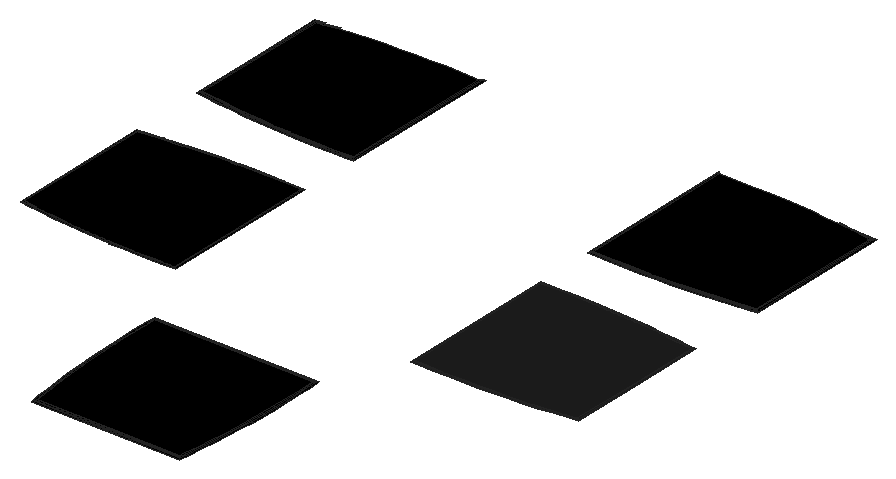
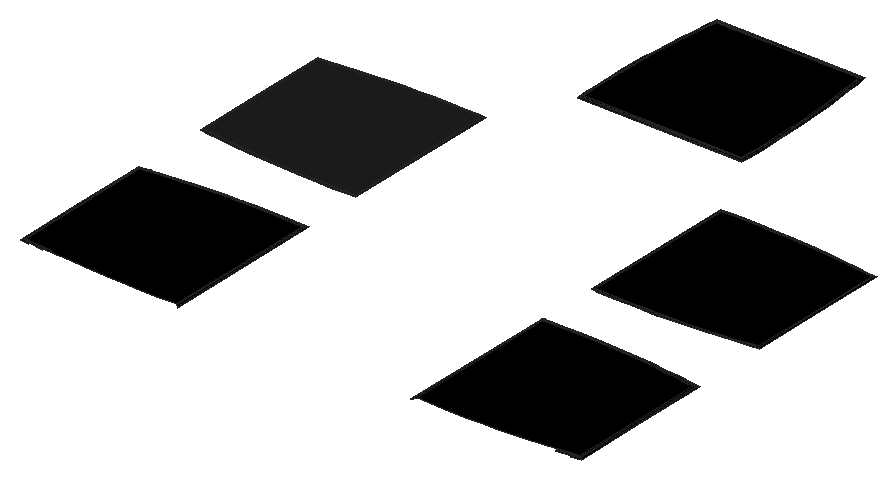
# SketchUp Ruby script. Lengths in inches.
U = 1.inch
M = Sketchup.active_model
def pt(a) = Geom::Point3d.new(a.map { |v| v * U })
def face(e, loops, mat)
  f = e.add_face(loops[0].map { |a| pt(a) })
  loops[1..].each { |l| e.add_face(l.map { |a| pt(a) }).erase! }
  f.material = f.back_material = mat if mat
  f
end
# faces: each face lists its corners as indices into pts; further lists are holes
def faces(e, pts, list, mat = nil) = list.each { |f| face(e, (f[0].is_a?(Array) ? f : [f]).map { |l| l.map { |i| pts[i] } }, mat) }
# xy, xz, yz: faces in a plane at the given z, y or x. An outline is a flat list of corners, or four numbers for a rectangle; further outlines are holes
def ring(l) = l.size == 4 ? [[l[0], l[1]], [l[2], l[1]], [l[2], l[3]], [l[0], l[3]]] : l.each_slice(2).to_a
def flat(e, list, mat, &to3) = list.each { |f| face(e, (f[0].is_a?(Array) ? f : [f]).map { |l| ring(l).map { |u, v| to3.(u, v) } }, mat) }
def xy(e, z, list, mat = nil) = flat(e, list, mat) { |x, y| [x, y, z] }
def xz(e, y, list, mat = nil) = flat(e, list, mat) { |x, z| [x, y, z] }
def yz(e, x, list, mat = nil) = flat(e, list, mat) { |y, z| [x, y, z] }
def lines(e, pts, list) = list.each { |a, b| e.add_line(pt(pts[a]), pt(pts[b])) }
# prism: a flat outline (further loops are holes) pulled along v
def prism(e, loops, v, mat = nil)
  f = face(e, loops, mat); d = Geom::Vector3d.new(v.map { |x| x * U })
  f.pushpull(f.normal.samedirection?(d) ? d.length : -d.length)
end
def box(e, o, s, mat = nil) = prism(e, [[o, [o[0] + s[0], o[1], o[2]], [o[0] + s[0], o[1] + s[1], o[2]], [o[0], o[1] + s[1], o[2]]]], [0, 0, s[2]], mat)
def at(x, y, z, deg = 0) = Geom::Transformation.translation(pt([x, y, z])) * Geom::Transformation.rotation(ORIGIN, Z_AXIS, deg.degrees)
def axes(o, x, y, z) = Geom::Transformation.new([*x, 0, *y, 0, *z, 0, *pt(o).to_a, 1])
def part(name) = M.definitions.add(name)
# library, detail: a bought-in or finely detailed component or shape, given as its bounding box
def library(name, o, s) = part(name).tap { |d| box(d.entities, o, s) }
def detail(e, o, s) = box(e.add_group.entities, o, s)
def put(e, d, t, mat = nil) = e.add_instance(d, t).tap { |i| i.material = mat if mat }
def group(e, t, mat = nil) = e.add_group.tap { |g| g.transformation = t; g.material = mat if mat }.entities
root = M.entities
M.materials.add("[Color M08]").color = [30, 30, 30]
M.materials.add("[Color M09]").color = [0, 0, 0]
xy(root,29.97,[[132.31,88.17,134,88.18,135.68,88.23,135.7,88.23,137.375,88.3,139.0625,88.39,140.75,88.52,142.43,88.68,144.1,88.86,145.78,89.07,146.49,89.17,146.49,105.6,145.78,105.7,144.1,105.91,142.43,106.09,140.75,106.24,139.0625,106.37,137.375,106.47,135.7,106.54,135.68,106.54,134,106.58,132.31,106.59,130.625,106.58,128.9375,106.54,128.32,106.51,128.32,88.25,128.9375,88.23,130.625,88.18]],"[Color M08]")
xy(root,29.97,[[106.15,61.21,122.58,61.21,122.68,61.92,122.89,63.6,123.07,65.28,123.22,66.96,123.35,68.64,123.45,70.33,123.52,72,123.52,72.02,123.56,73.7,123.57,75.39,123.56,77.08,123.52,78.76,123.49,79.38,105.23,79.38,105.21,78.76,105.16,77.08,105.15,75.39,105.16,73.7,105.21,72.02,105.21,72,105.28,70.33,105.375,68.64,105.5,66.96,105.65,65.28,105.84,63.6,106.05,61.92],[96.41,88.17,98.1,88.18,99.78,88.23,100.4,88.25,100.4,106.51,99.78,106.54,98.1,106.58,96.41,106.59,94.72,106.58,93.04,106.54,93.02,106.54,91.35,106.47,89.66,106.37,87.98,106.24,86.3,106.09,84.62,105.91,82.94,105.7,82.23,105.6,82.23,89.17,82.94,89.07,84.62,88.86,86.3,88.68,87.98,88.52,89.66,88.39,91.35,88.3,93.02,88.23,93.04,88.23,94.72,88.18],[96.41,114.08,98.1,114.09,99.78,114.13,100.4,114.16,100.4,132.42,99.78,132.44,98.1,132.49,96.41,132.5,94.72,132.49,93.04,132.44,93.02,132.44,91.35,132.375,89.66,132.28,87.98,132.15,86.3,132,84.62,131.8125,82.94,131.6,82.23,131.5,82.23,115.07,82.94,114.97,84.62,114.76,86.3,114.58,87.98,114.43,89.66,114.3,91.35,114.2,93.02,114.13,93.04,114.13,94.72,114.09],[132.31,114.08,134,114.09,135.68,114.13,135.7,114.13,137.375,114.2,139.0625,114.3,140.75,114.43,142.43,114.58,144.1,114.76,145.78,114.97,146.49,115.07,146.49,131.5,145.78,131.6,144.1,131.8125,142.43,132,140.75,132.15,139.0625,132.28,137.375,132.375,135.7,132.44,135.68,132.44,134,132.49,132.31,132.5,130.625,132.49,128.9375,132.44,128.32,132.42,128.32,114.16,128.9375,114.13,130.625,114.09]],"[Color M09]")
p = [[105.76,61.89,29.93],[105.62,61.87,29.89],[105.77,60.78,29.89],[105.9,60.92,29.93],[114.36,60.78,29.89],[114.36,60.92,29.93],
  [122.95,60.78,29.89],[122.83,60.92,29.93],[123.1,61.87,29.89],[122.97,61.89,29.93],[105.9,61.9,29.96],[106.02,61.0625,29.96],
  [114.36,61.0625,29.96],[122.7,61.0625,29.96],[122.82,61.9,29.96],[105.55,63.57,29.93],[105.41,63.55,29.89],[105.69,63.58,29.96],
  [123.18,63.57,29.93],[123.03,63.58,29.96],[123.3125,63.55,29.89],[105.37,65.25,29.93],[105.23,65.23,29.89],[123.5,65.23,29.89],
  [123.36,65.25,29.93],[105.51,65.26,29.96],[123.21,65.26,29.96],[105.21,66.93,29.93],[105.07,66.92,29.89],[105.35,66.95,29.96],
  [123.51,66.93,29.93],[123.37,66.95,29.96],[123.65,66.92,29.89],[105.08,68.62,29.93],[104.94,68.61,29.89],[105.23,68.63,29.96],
  [123.64,68.62,29.93],[123.5,68.63,29.96],[123.78,68.61,29.89],[104.99,70.3125,29.93],[104.85,70.31,29.89],[105.13,70.32,29.96],
  [123.74,70.3125,29.93],[123.59,70.32,29.96],[123.88,70.31,29.89],[104.78,71.99,29.89],[104.91,72,29.93],[105.06,72,29.96],
  [123.81,72,29.93],[123.66,72,29.96],[123.95,71.99,29.89],[104.78,72.01,29.89],[104.73,73.69,29.89],[104.87,73.7,29.93],
  [104.91,72.01,29.93],[105.06,72.02,29.96],[105.02,73.7,29.96],[123.67,72.02,29.96],[123.81,72.01,29.93],[123.85,73.7,29.93],
  [123.71,73.7,29.96],[123.95,72.01,29.89],[123.99,73.69,29.89],[104.72,75.39,29.89],[104.86,75.39,29.93],[105,75.39,29.96],
  [123.72,75.39,29.96],[123.87,75.39,29.93],[124,75.39,29.89],[104.73,77.08,29.89],[104.87,77.08,29.93],[105.02,77.08,29.96],
  [123.71,77.08,29.96],[123.85,77.08,29.93],[123.99,77.08,29.89],[104.77,78.78,29.89],[104.91,78.77,29.93],[105.06,78.77,29.96],
  [123.67,78.77,29.96],[123.81,78.77,29.93],[123.95,78.78,29.89],[104.82,79.8125,29.89],[104.95,79.67,29.93],[105.09,79.53,29.96],
  [123.63,79.53,29.96],[123.77,79.67,29.93],[123.91,79.8125,29.89],[91.33,88.01,29.93],[93.02,87.94,29.93],[93.02,88.08,29.96],
  [91.34,88.15,29.96],[94.72,87.89,29.93],[93.03,87.93,29.93],[93.04,88.08,29.96],[94.72,88.04,29.96],[96.41,88.02,29.96],
  [96.41,87.88,29.93],[98.1,88.04,29.96],[98.1,87.89,29.93],[99.79,88.08,29.96],[99.79,87.93,29.93],[100.55,88.11,29.96],
  [100.69,87.97,29.93],[128.93,88.08,29.96],[128.93,87.93,29.93],[128.03,87.97,29.93],[128.18,88.11,29.96],[130.625,88.04,29.96],
  [130.62,87.89,29.93],[132.31,88.02,29.96],[132.31,87.88,29.93],[134.01,88.04,29.96],[134.01,87.89,29.93],[135.69,87.93,29.93],
  [135.6875,88.08,29.96],[135.7,88.08,29.96],[135.71,87.94,29.93],[137.39,88.01,29.93],[137.38,88.15,29.96],[89.65,88.25,29.96],
  [89.64,88.1,29.93],[100.55,106.65,29.96],[100.69,106.79,29.93],[128.03,106.79,29.93],[128.18,106.65,29.96],[139.08,88.1,29.93],
  [139.07,88.25,29.96],[87.97,88.375,29.96],[87.95,88.23,29.93],[140.77,88.23,29.93],[140.76,88.375,29.96],[86.28,88.53,29.96],
  [86.27,88.39,29.93],[142.46,88.39,29.93],[142.44,88.53,29.96],[84.6,88.71,29.96],[84.59,88.57,29.93],[144.14,88.57,29.93],
  [144.12,88.71,29.96],[82.92,88.92,29.96],[82.91,88.78,29.93],[145.82,88.78,29.93],[145.8,88.92,29.96],[82.08,89.04,29.96],
  [81.9375,88.92,29.93],[146.78,88.92,29.93],[146.64,89.04,29.96],[82.08,97.38,29.96],[81.9375,97.38,29.93],[146.78,97.38,29.93],
  [146.64,97.38,29.96],[82.08,105.72,29.96],[81.9375,105.85,29.93],[146.78,105.85,29.93],[146.64,105.72,29.96],[82.92,105.84,29.96],
  [82.91,105.99,29.93],[145.82,105.99,29.93],[145.8,105.84,29.96],[84.6,106.05,29.96],[84.59,106.2,29.93],[144.14,106.2,29.93],
  [144.12,106.05,29.96],[86.28,106.24,29.96],[86.27,106.38,29.93],[142.46,106.38,29.93],[142.44,106.24,29.96],[87.97,106.39,29.96],
  [87.95,106.53,29.93],[140.77,106.53,29.93],[140.76,106.39,29.96],[89.65,106.52,29.96],[89.64,106.66,29.93],[139.08,106.66,29.93],
  [139.07,106.52,29.96],[91.34,106.61,29.96],[91.33,106.76,29.93],[137.39,106.76,29.93],[137.38,106.61,29.96],[93.02,106.83,29.93],
  [93.02,106.68,29.96],[135.71,106.83,29.93],[135.7,106.68,29.96],[93.04,106.6875,29.96],[93.03,106.83,29.93],[94.72,106.87,29.93],
  [94.72,106.73,29.96],[96.41,106.89,29.93],[96.41,106.74,29.96],[98.1,106.87,29.93],[98.1,106.73,29.96],[99.79,106.83,29.93],
  [99.79,106.6875,29.96],[128.93,106.83,29.93],[128.93,106.6875,29.96],[130.62,106.87,29.93],[130.625,106.73,29.96],[132.31,106.89,29.93],
  [132.31,106.74,29.96],[134.01,106.87,29.93],[134.01,106.73,29.96],[135.69,106.83,29.93],[135.6875,106.6875,29.96],[94.71,113.66,29.89],
  [94.72,113.8,29.93],[96.41,113.78,29.93],[96.41,113.65,29.89],[98.1,113.8,29.93],[98.1,113.66,29.89],[132.31,113.78,29.93],
  [132.31,113.65,29.89],[130.62,113.66,29.89],[130.62,113.8,29.93],[134.01,113.8,29.93],[134.01,113.66,29.89],[91.33,113.77,29.89],
  [93.01,113.7,29.89],[93.02,113.84,29.93],[91.33,113.91,29.93],[93.02,113.7,29.89],[93.03,113.84,29.93],[99.79,113.84,29.93],
  [99.8,113.7,29.89],[100.69,113.88,29.93],[100.83,113.74,29.89],[100.69,132.7,29.93],[100.83,132.83,29.89],[128.93,113.84,29.93],
  [128.92,113.7,29.89],[127.89,113.74,29.89],[128.03,113.88,29.93],[127.89,132.83,29.89],[128.03,132.7,29.93],[135.7,113.7,29.89],
  [135.69,113.84,29.93],[135.71,113.84,29.93],[135.71,113.7,29.89],[137.4,113.77,29.89],[137.39,113.91,29.93],[89.64,114.01,29.93],
  [89.63,113.87,29.89],[93.02,113.99,29.96],[91.34,114.06,29.96],[93.04,113.98,29.96],[94.72,113.94,29.96],[96.41,113.93,29.96],
  [98.1,113.94,29.96],[99.79,113.98,29.96],[100.55,114.02,29.96],[128.93,113.98,29.96],[128.18,114.02,29.96],[130.625,113.94,29.96],
  [132.31,113.93,29.96],[134.01,113.94,29.96],[135.6875,113.98,29.96],[135.7,113.99,29.96],[137.38,114.06,29.96],[139.09,113.87,29.89],
  [139.08,114.01,29.93],[87.95,114.14,29.93],[87.94,114,29.89],[89.65,114.15,29.96],[100.55,132.56,29.96],[128.18,132.56,29.96],
  [139.07,114.15,29.96],[140.78,114,29.89],[140.77,114.14,29.93],[86.27,114.29,29.93],[86.25,114.15,29.89],[87.97,114.28,29.96],
  [140.76,114.28,29.96],[142.47,114.15,29.89],[142.46,114.29,29.93],[86.28,114.44,29.96],[142.44,114.44,29.96],[84.59,114.47,29.93],
  [84.57,114.34,29.89],[144.15,114.34,29.89],[144.14,114.47,29.93],[82.91,114.68,29.93],[82.89,114.55,29.89],[84.6,114.62,29.96],
  [144.12,114.62,29.96],[145.84,114.55,29.89],[145.82,114.68,29.93],[81.9375,114.82,29.93],[81.8,114.7,29.89],[82.92,114.83,29.96],
  [145.8,114.83,29.96],[146.92,114.7,29.89],[146.78,114.82,29.93],[81.9375,123.29,29.93],[81.8,123.29,29.89],[82.08,114.95,29.96],
  [146.64,114.95,29.96],[146.92,123.29,29.89],[146.78,123.29,29.93],[82.08,123.29,29.96],[146.64,123.29,29.96],[81.9375,131.75,29.93],
  [81.8,131.875,29.89],[82.08,131.63,29.96],[146.78,131.75,29.93],[146.64,131.63,29.96],[146.92,131.875,29.89],[82.92,131.75,29.96],
  [82.91,131.89,29.93],[145.82,131.89,29.93],[145.8,131.75,29.96],[84.6,131.96,29.96],[84.59,132.1,29.93],[144.14,132.1,29.93],
  [144.12,131.96,29.96],[82.89,132.03,29.89],[145.84,132.03,29.89],[106.05,61.92,29.97],[106.15,61.21,29.97],[114.36,61.21,29.97],
  [122.58,61.21,29.97],[122.68,61.92,29.97],[105.84,63.6,29.97],[122.89,63.6,29.97],[105.65,65.28,29.97],[123.07,65.28,29.97],
  [105.5,66.96,29.97],[123.22,66.96,29.97],[105.375,68.64,29.97],[123.35,68.64,29.97],[105.28,70.33,29.97],[123.45,70.33,29.97],
  [105.21,72,29.97],[123.52,72,29.97],[105.16,73.7,29.97],[105.21,72.02,29.97],[123.52,72.02,29.97],[123.56,73.7,29.97],
  [105.15,75.39,29.97],[123.57,75.39,29.97],[105.16,77.08,29.97],[123.56,77.08,29.97],[105.21,78.76,29.97],[123.52,78.76,29.97],
  [105.23,79.38,29.97],[123.49,79.38,29.97],[93.04,88.23,29.97],[94.72,88.18,29.97],[96.41,88.17,29.97],[98.1,88.18,29.97],
  [99.78,88.23,29.97],[130.625,88.18,29.97],[128.9375,88.23,29.97],[132.31,88.17,29.97],[134,88.18,29.97],[135.68,88.23,29.97],
  [91.35,88.3,29.97],[89.66,88.39,29.97],[93.02,88.23,29.97],[100.4,88.25,29.97],[100.4,106.51,29.97],[128.32,88.25,29.97],
  [128.32,106.51,29.97],[135.7,88.23,29.97],[137.375,88.3,29.97],[139.0625,88.39,29.97],[87.98,88.52,29.97],[140.75,88.52,29.97],
  [86.3,88.68,29.97],[142.43,88.68,29.97],[84.62,88.86,29.97],[144.1,88.86,29.97],[82.94,89.07,29.97],[145.78,89.07,29.97],
  [82.23,89.17,29.97],[146.49,89.17,29.97],[82.23,97.38,29.97],[146.49,97.38,29.97],[82.23,105.6,29.97],[146.49,105.6,29.97],
  [82.94,105.7,29.97],[145.78,105.7,29.97],[84.62,105.91,29.97],[144.1,105.91,29.97],[86.3,106.09,29.97],[142.43,106.09,29.97],
  [87.98,106.24,29.97],[140.75,106.24,29.97],[89.66,106.37,29.97],[139.0625,106.37,29.97],[91.35,106.47,29.97],[137.375,106.47,29.97],
  [93.02,106.54,29.97],[93.04,106.54,29.97],[94.72,106.58,29.97],[98.1,106.58,29.97],[99.78,106.54,29.97],[128.9375,106.54,29.97],
  [130.625,106.58,29.97],[135.68,106.54,29.97],[134,106.58,29.97],[135.7,106.54,29.97],[96.41,106.59,29.97],[132.31,106.59,29.97],
  [93.04,114.13,29.97],[94.72,114.09,29.97],[96.41,114.08,29.97],[98.1,114.09,29.97],[99.78,114.13,29.97],[130.625,114.09,29.97],
  [128.9375,114.13,29.97],[132.31,114.08,29.97],[134,114.09,29.97],[135.68,114.13,29.97],[93.02,114.13,29.97],[91.35,114.2,29.97],
  [100.4,114.16,29.97],[100.4,132.42,29.97],[128.32,114.16,29.97],[128.32,132.42,29.97],[135.7,114.13,29.97],[137.375,114.2,29.97],
  [89.66,114.3,29.97],[139.0625,114.3,29.97],[87.98,114.43,29.97],[140.75,114.43,29.97],[86.3,114.58,29.97],[142.43,114.58,29.97],
  [84.62,114.76,29.97],[144.1,114.76,29.97],[82.94,114.97,29.97],[145.78,114.97,29.97],[82.23,115.07,29.97],[146.49,115.07,29.97],
  [82.23,123.29,29.97],[146.49,123.29,29.97],[82.23,131.5,29.97],[146.49,131.5,29.97],[82.94,131.6,29.97],[145.78,131.6,29.97],
  [84.62,131.8125,29.97],[144.1,131.8125,29.97],[142.44,132.14,29.96],[142.43,132,29.97]]
faces(root,p,[[0,1,2,3],[3,2,4,5],[6,7,5,4],[8,9,7,6],[10,0,3,11],[11,3,5,12],[7,13,12,5],[9,14,13,7],
  [15,16,1,0],[17,15,0,10],[18,19,14,9],[20,18,9,8],[21,22,16,15],[23,24,18,20],[25,21,15,17],[24,26,19,18],
  [27,28,22,21],[29,27,21,25],[30,31,26,24],[32,30,24,23],[33,34,28,27],[35,33,27,29],[36,37,31,30],[38,36,30,32],
  [39,40,34,33],[41,39,33,35],[42,43,37,36],[44,42,36,38],[45,40,39,46],[46,39,41,47],[42,48,49,43],[44,50,48,42],
  [51,52,53,54],[54,46,45,51],[55,47,46,54],[54,53,56,55],[57,49,48,58],[59,58,57,60],[58,48,50,61],[62,61,58,59],
  [53,52,63,64],[56,53,64,65],[59,60,66,67],[62,59,67,68],[64,63,69,70],[65,64,70,71],[67,66,72,73],[68,67,73,74],
  [70,69,75,76],[71,70,76,77],[73,72,78,79],[74,73,79,80],[76,75,81,82],[77,76,82,83],[79,78,84,85],[80,79,85,86],
  [83,82,85,84],[82,81,86,85],[87,88,89,90],[91,92,93,94],[93,89,88,92],[91,94,95,96],[96,95,97,98],[98,97,99,100],
  [100,99,101,102],[87,90,119,120],[121,122,102,101],[120,119,127,128],[128,127,131,132],[132,131,135,136],[136,135,139,140],[140,139,143,144],
  [144,143,147,148],[151,152,148,147],[155,156,152,151],[159,160,156,155],[163,164,160,159],[167,168,164,163],[171,172,168,167],[175,176,172,171],
  [179,176,175,180],[183,180,179,184],[184,185,186,183],[186,185,187,188],[188,187,189,190],[190,189,191,192],[192,191,122,121],[203,204,205,206],
  [206,205,207,208],[209,210,211,212],[213,214,210,209],[215,216,217,218],[203,219,220,204],[220,217,216,219],[208,207,221,222],[222,221,223,224],
  [225,226,224,223],[227,228,229,230],[230,229,231,232],[212,211,228,227],[233,214,213,234],[234,235,236,233],[236,237,238,235],[215,218,239,240],
  [218,217,241,242],[204,220,243,244],[243,241,217,220],[204,244,245,205],[205,245,246,207],[207,246,247,221],[221,247,248,223],[249,227,230,250],
  [251,212,227,249],[252,209,212,251],[253,213,209,252],[234,213,253,254],[254,255,235,234],[235,238,256,255],[238,237,257,258],[240,239,259,260],
  [218,242,261,239],[262,225,223,248],[250,230,232,263],[256,238,258,264],[258,257,265,266],[260,259,267,268],[239,261,269,259],[264,258,266,270],
  [266,265,271,272],[259,269,273,267],[270,266,272,274],[268,267,275,276],[272,271,277,278],[276,275,279,280],[267,273,281,275],[274,272,278,282],
  [278,277,283,284],[280,279,285,286],[275,281,287,279],[282,278,284,288],[284,283,289,290],[286,285,291,292],[279,287,293,285],[288,284,290,294],
  [290,289,295,296],[285,293,297,291],[294,290,296,298],[299,300,292,291],[301,299,291,297],[302,303,298,296],[304,302,296,295],[305,306,299,301],
  [307,308,303,302],[309,310,306,305],[311,312,308,307],[306,313,300,299],[314,307,302,304],[315,10,11,316],[316,11,12,317],[13,318,317,12],
  [14,319,318,13],[320,17,10,315],[19,321,319,14],[322,25,17,320],[26,323,321,19],[324,29,25,322],[31,325,323,26],[326,35,29,324],
  [37,327,325,31],[328,41,35,326],[43,329,327,37],[47,41,328,330],[43,49,331,329],[55,56,332,333],[333,330,47,55],[334,331,49,57],
  [60,57,334,335],[332,56,65,336],[60,335,337,66],[336,65,71,338],[66,337,339,72],[338,71,77,340],[72,339,341,78],[340,77,83,342],
  [78,341,343,84],[342,83,84,343],[94,93,344,345],[94,345,346,95],[95,346,347,97],[97,347,348,99],[90,354,355,119],[90,89,356,354],
  [344,356,89,93],[99,348,357,101],[358,121,101,357],[119,355,364,127],[127,364,366,131],[131,366,368,135],[135,368,370,139],[139,370,372,143],
  [143,372,374,147],[376,151,147,374],[378,155,151,376],[380,159,155,378],[382,163,159,380],[384,167,163,382],[386,171,167,384],[388,175,171,386],
  [180,175,388,390],[391,390,180,183],[183,186,392,391],[393,190,192,394],[394,192,121,358],[392,186,188,400],[400,188,190,393],[244,243,402,403],
  [244,403,404,245],[245,404,405,246],[246,405,406,247],[407,251,249,408],[409,252,251,407],[410,253,252,409],[254,253,410,411],[242,241,412,413],
  [402,412,241,243],[247,406,414,248],[415,262,248,414],[408,249,250,416],[416,250,263,417],[411,418,255,254],[255,256,419,418],[242,413,420,261],
  [419,256,264,421],[261,420,422,269],[421,264,270,423],[269,422,424,273],[423,270,274,425],[273,424,426,281],[425,274,282,427],[281,426,428,287],
  [427,282,288,429],[287,428,430,293],[429,288,294,431],[293,430,432,297],[431,294,298,433],[434,301,297,432],[303,435,433,298],[436,305,301,434],
  [308,437,435,303],[438,309,305,436],[312,439,437,308],[440,441,439,312]],"[Color M09]")
faces(root,p,[[103,104,105,106],[107,108,104,103],[109,110,108,107],[111,112,110,109],[113,112,111,114],[114,115,116,113],[116,117,118,115],[106,105,123,124],
  [118,117,125,126],[126,125,129,130],[130,129,133,134],[134,133,137,138],[138,137,141,142],[142,141,145,146],[146,145,149,150],[153,154,150,149],
  [157,158,154,153],[161,162,158,157],[165,166,162,161],[169,170,166,165],[173,174,170,169],[177,178,174,173],[177,181,182,178],[193,194,124,123],
  [195,196,194,193],[197,198,196,195],[199,200,198,197],[199,201,202,200],[202,182,181,201],[349,107,103,350],[351,109,107,349],[352,111,109,351],
  [114,111,352,353],[350,103,106,359],[359,106,124,360],[353,361,115,114],[115,118,362,361],[362,118,126,363],[363,126,130,365],[365,130,134,367],
  [367,134,138,369],[369,138,142,371],[371,142,146,373],[373,146,150,375],[154,377,375,150],[158,379,377,154],[162,381,379,158],[166,383,381,162],
  [170,385,383,166],[174,387,385,170],[178,389,387,174],[194,395,360,124],[196,396,395,194],[200,202,397,398],[178,182,399,389],[397,399,182,202],
  [198,401,396,196],[200,398,401,198]],"[Color M08]")
